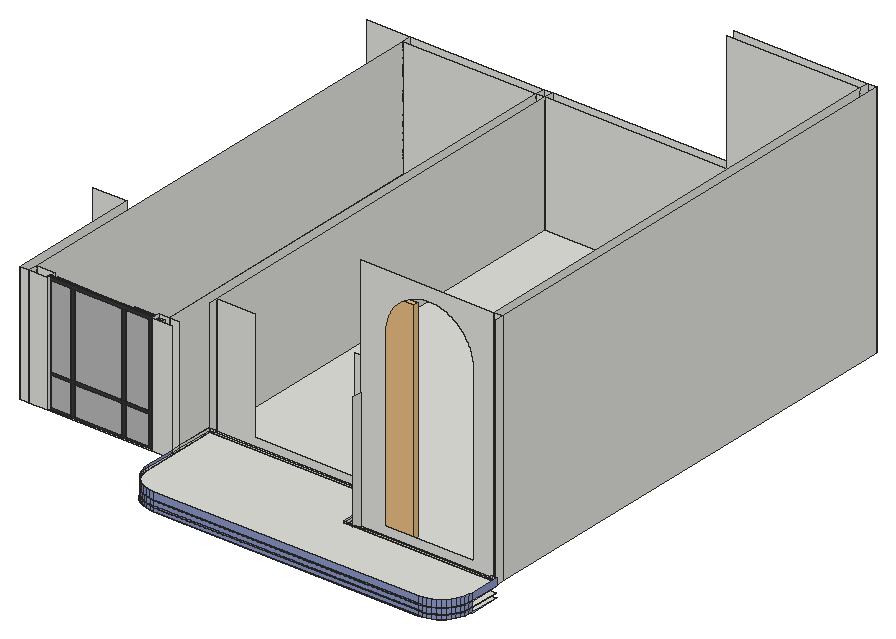
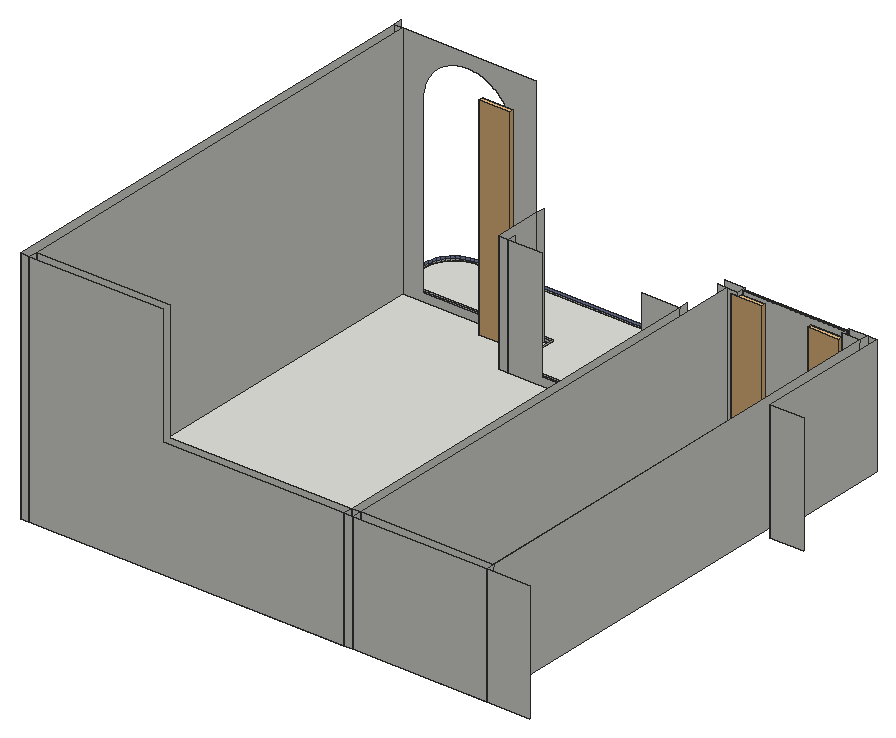
# SketchUp Ruby script. Lengths in inches.
U = 1.inch
M = Sketchup.active_model
def pt(a) = Geom::Point3d.new(a.map { |v| v * U })
def face(e, loops, mat)
  f = e.add_face(loops[0].map { |a| pt(a) })
  loops[1..].each { |l| e.add_face(l.map { |a| pt(a) }).erase! }
  f.material = f.back_material = mat if mat
  f
end
# faces: each face lists its corners as indices into pts; further lists are holes
def faces(e, pts, list, mat = nil) = list.each { |f| face(e, (f[0].is_a?(Array) ? f : [f]).map { |l| l.map { |i| pts[i] } }, mat) }
# xy, xz, yz: faces in a plane at the given z, y or x. An outline is a flat list of corners, or four numbers for a rectangle; further outlines are holes
def ring(l) = l.size == 4 ? [[l[0], l[1]], [l[2], l[1]], [l[2], l[3]], [l[0], l[3]]] : l.each_slice(2).to_a
def flat(e, list, mat, &to3) = list.each { |f| face(e, (f[0].is_a?(Array) ? f : [f]).map { |l| ring(l).map { |u, v| to3.(u, v) } }, mat) }
def xy(e, z, list, mat = nil) = flat(e, list, mat) { |x, y| [x, y, z] }
def xz(e, y, list, mat = nil) = flat(e, list, mat) { |x, z| [x, y, z] }
def yz(e, x, list, mat = nil) = flat(e, list, mat) { |y, z| [x, y, z] }
def lines(e, pts, list) = list.each { |a, b| e.add_line(pt(pts[a]), pt(pts[b])) }
# prism: a flat outline (further loops are holes) pulled along v
def prism(e, loops, v, mat = nil)
  f = face(e, loops, mat); d = Geom::Vector3d.new(v.map { |x| x * U })
  f.pushpull(f.normal.samedirection?(d) ? d.length : -d.length)
end
def box(e, o, s, mat = nil) = prism(e, [[o, [o[0] + s[0], o[1], o[2]], [o[0] + s[0], o[1] + s[1], o[2]], [o[0], o[1] + s[1], o[2]]]], [0, 0, s[2]], mat)
def at(x, y, z, deg = 0) = Geom::Transformation.translation(pt([x, y, z])) * Geom::Transformation.rotation(ORIGIN, Z_AXIS, deg.degrees)
def axes(o, x, y, z) = Geom::Transformation.new([*x, 0, *y, 0, *z, 0, *pt(o).to_a, 1])
def part(name) = M.definitions.add(name)
# library, detail: a bought-in or finely detailed component or shape, given as its bounding box
def library(name, o, s) = part(name).tap { |d| box(d.entities, o, s) }
def detail(e, o, s) = box(e.add_group.entities, o, s)
def put(e, d, t, mat = nil) = e.add_instance(d, t).tap { |i| i.material = mat if mat }
def group(e, t, mat = nil) = e.add_group.tap { |g| g.transformation = t; g.material = mat if mat }.entities
root = M.entities
M.materials.add("0326 AP 7207 CLASSIC PURPLE").color = [140, 152, 201]
M.materials.add("[Color M07]").color = [58, 58, 58]
M.materials.add("[Mirror 01]").color = [185, 185, 185]
c1 = library("Curtains 004",[-15.59,-2.26,0],[31.18,4.52,116.91])
xy(root,120.625,[[220.41,30.14,217,30.36,213.65,31.03,210.41,32.125,207.35,33.64,204.51,35.53,201.94,37.79,199.69,40.35,197.79,43.19,196.28,46.26,195.18,49.49,194.52,52.84,194.29,56.25,194.29,109.85,196.02,109.85,196.02,56.25,196.23,53.07,196.85,49.9375,197.88,46.92,199.29,44.06,201.0625,41.41,203.16,39.01,205.5625,36.9,208.21,35.13,211.08,33.72,214.1,32.7,217.22,32.07,220.41,31.87,487.22,31.87,490.59,32.09,493.71,32.71,496.73,33.73,499.59,35.14,502.24,36.91,504.64,39.02,506.74,41.41,508.51,44.0625,509.92,46.92,510.95,49.94,511.57,53.07,511.79,56.43,511.79,86.25,513.52,86.25,513.52,56.38,513.29,52.84,512.62,49.49,511.52,46.26,510.01,43.2,508.12,40.36,505.87,37.79,505.84,37.77,503.3,35.54,500.46,33.64,497.4,32.13,494.16,31.03,490.8125,30.37,487.28,30.14]])
xy(root,120.9375,[[220.41,29.57,216.92,29.79,213.5,30.47,210.2,31.6,207.06,33.14,204.16,35.08,201.54,37.38,199.24,40.01,197.3,42.91,195.75,46.04,194.63,49.34,193.95,52.77,193.72,56.25,193.72,109.85,196.02,109.85,196.02,56.25,196.23,53.07,196.85,49.9375,197.88,46.92,199.29,44.06,201.0625,41.41,203.16,39.01,205.5625,36.9,208.21,35.13,211.08,33.72,214.1,32.7,217.22,32.07,220.41,31.87,487.22,31.87,490.59,32.09,493.71,32.71,496.73,33.73,499.59,35.14,502.24,36.91,504.64,39.02,506.74,41.41,508.51,44.0625,509.92,46.92,510.95,49.94,511.57,53.07,511.79,56.43,511.79,86.25,514.09,86.25,514.09,56.36,513.86,52.77,513.18,49.35,512.05,46.04,510.51,42.91,508.57,40.01,506.27,37.39,506.22,37.34,503.65,35.09,500.75,33.15,497.62,31.6,494.3125,30.48,490.89,29.8,487.3,29.57]])
xy(root,121.1875,[[220.41,26.25,487.41,26.25,491.32,26.51,495.17,27.27,498.89,28.53,502.41,30.27,505.67,32.45,508.41,34.85,508.62,35.04,511.21,37.99,513.39,41.25,515.125,44.77,516.38,48.49,517.15,52.33,517.41,56.25,517.41,86.25,364.41,86.25,364.41,133.75,190.41,133.75,190.41,56.25,190.66,52.33,191.43,48.49,192.69,44.77,194.43,41.25,196.61,37.99,199.19,35.04,202.14,32.45,205.41,30.27,208.93,28.53,212.64,27.27,216.49,26.51]])
xy(root,121.1875,[[220.41,25.68,487.43,25.68,491.4,25.9375,495.32,26.72,499.11,28,502.69,29.77,506.02,32,508.78,34.42,509.02,34.63,511.66,37.64,513.88,40.96,515.65,44.55,516.9375,48.34,517.72,52.26,517.98,56.23,517.98,86.82,517.41,86.82,517.41,56.25,517.15,52.33,516.38,48.49,515.125,44.77,513.39,41.25,511.21,37.99,508.62,35.04,508.41,34.85,505.67,32.45,502.41,30.27,498.89,28.53,495.17,27.27,491.32,26.51,487.41,26.25,220.41,26.25,216.49,26.51,212.64,27.27,208.93,28.53,205.41,30.27,202.14,32.45,199.19,35.04,196.61,37.99,194.43,41.25,192.69,44.77,191.43,48.49,190.66,52.33,190.41,56.25,190.41,86.25,189.84,86.25,189.84,56.25,190.1,52.26,190.88,48.34,192.16,44.55,193.93,40.96,196.15,37.64,198.79,34.63,201.8,32,205.12,29.77,208.71,28.01,212.49,26.72,216.42,25.94]],"0326 AP 7207 CLASSIC PURPLE")
xy(root,124.75,[[220.41,26.25,487.41,26.25,491.32,26.51,495.17,27.27,498.89,28.53,502.41,30.27,505.67,32.45,508.62,35.04,511.21,37.99,513.39,41.25,515.125,44.77,516.38,48.49,517.15,52.33,517.41,56.25,517.41,86.25,364.41,86.25,364.41,133.75,190.41,133.75,190.41,56.25,190.66,52.33,191.43,48.49,192.69,44.77,194.43,41.25,196.61,37.99,199.19,35.04,202.14,32.45,205.41,30.27,208.93,28.53,212.64,27.27,216.49,26.51]])
xy(root,125.8125,[[220.41,26.25,487.41,26.25,491.32,26.51,495.17,27.27,498.89,28.53,502.41,30.27,505.67,32.45,508.62,35.04,511.21,37.99,513.39,41.25,515.125,44.77,516.38,48.49,517.15,52.33,517.41,56.25,517.41,86.25,364.41,86.25,364.41,133.75,190.41,133.75,190.41,56.25,190.66,52.33,191.43,48.49,192.69,44.77,194.43,41.25,196.61,37.99,199.19,35.04,202.14,32.45,205.41,30.27,208.93,28.53,212.64,27.27,216.49,26.51]])
xy(root,130.64,[[63.57,88.4,168.59,90.22]],"[Color M07]")
xy(root,130.9375,[[220.41,26.25,487.41,26.25,491.32,26.51,495.17,27.27,498.89,28.53,502.41,30.27,505.67,32.45,508.62,35.04,511.21,37.99,513.39,41.25,515.125,44.77,516.38,48.49,517.15,52.33,517.41,56.25,517.41,86.25,364.41,86.25,364.41,133.75,190.41,133.75,190.41,56.25,190.66,52.33,191.43,48.49,192.69,44.77,194.43,41.25,196.61,37.99,199.19,35.04,202.14,32.45,205.41,30.27,208.93,28.53,212.64,27.27,216.49,26.51]])
xy(root,132,[[46.41,86.25,65.51,95.25],[65.51,86.25,169.65,95.25],[169.65,86.25,190.41,95.25],[364.41,86.25,373.41,142.75],[373.41,86.25,517.41,95.25],
  [46.41,95.25,181.41,557.25],[181.41,95.25,190.41,557.25],[373.41,95.25,508.41,95.25,508.41,557.25,190.41,557.25,190.41,142.75,373.41,142.75],[508.41,95.25,517.41,566.25],[190.41,133.75,364.41,142.75],
  [46.41,557.25,181.41,566.25],[181.41,557.25,190.41,566.25],[190.41,557.25,508.41,566.25]])
xy(root,132.125,[[220.41,25.95,216.45,26.21,212.5625,26.98,208.81,28.25,205.26,30.01,201.96,32.21,198.98,34.82,196.37,37.8,194.16,41.1,192.41,44.65,191.14,48.41,190.36,52.29,190.1,56.25,190.1,134.05,195.11,134.05,195.11,133.75,190.41,133.75,190.41,56.25,190.66,52.33,191.43,48.49,192.69,44.77,194.43,41.25,196.61,37.99,199.19,35.04,202.14,32.45,205.41,30.27,208.93,28.53,212.64,27.27,216.49,26.51,220.41,26.25,487.41,26.25,491.32,26.51,495.17,27.27,498.89,28.53,502.41,30.27,505.67,32.45,508.62,35.04,511.21,37.99,513.39,41.25,515.125,44.77,516.38,48.49,517.15,52.33,517.41,56.25,517.41,86.25,512.71,86.25,512.71,86.55,517.71,86.55,517.71,56.25,517.45,52.29,516.68,48.41,515.4,44.65,513.65,41.1,511.45,37.8,508.83,34.82,505.85,32.21,502.56,30.01,499,28.25,495.25,26.98,491.36,26.21,487.41,25.95]],"0326 AP 7207 CLASSIC PURPLE")
xy(root,132.1875,[[220.41,26.25,487.41,26.25,491.32,26.51,495.17,27.27,498.89,28.53,502.41,30.27,505.67,32.45,508.62,35.04,511.21,37.99,513.39,41.25,515.125,44.77,516.38,48.49,517.15,52.33,517.41,56.25,517.41,86.25,364.41,86.25,364.41,133.75,190.41,133.75,190.41,56.25,190.66,52.33,191.43,48.49,192.69,44.77,194.43,41.25,196.61,37.99,199.19,35.04,202.14,32.45,205.41,30.27,208.93,28.53,212.64,27.27,216.49,26.51]])
xy(root,133.36,[[66.28,88.4,86.85,88.84],[90.47,88.4,138.0625,88.84],[142.18,88.4,165.87,88.84]],"[Color M07]")
xy(root,135.3125,[[220.41,26.25,487.41,26.25,491.32,26.51,495.17,27.27,498.89,28.53,502.41,30.27,505.67,32.45,508.62,35.04,511.21,37.99,513.39,41.25,515.125,44.77,516.38,48.49,517.15,52.33,517.41,56.25,517.41,86.25,364.41,86.25,364.41,133.75,190.41,133.75,190.41,56.25,190.66,52.33,191.43,48.49,192.69,44.77,194.43,41.25,196.61,37.99,199.19,35.04,202.14,32.45,205.41,30.27,208.93,28.53,212.64,27.27,216.49,26.51]])
xy(root,163.14,[[66.28,88.4,86.85,88.84],[90.47,88.4,138.0625,88.84],[142.18,88.4,165.87,88.84]],"[Color M07]")
xy(root,165.91,[[66.28,88.4,86.85,88.84],[90.47,88.4,138.0625,88.84],[142.18,88.4,165.87,88.84]],"[Color M07]")
xy(root,248.8,[[66.28,88.4,86.85,88.84],[90.47,88.4,138.0625,88.84],[142.18,88.4,165.87,88.84]],"[Color M07]")
xy(root,251.52,[[63.57,88.4,168.59,90.22]],"[Color M07]")
xz(root,25.95,[[220.41,132.125,487.41,139.125]],"0326 AP 7207 CLASSIC PURPLE")
xz(root,26.25,[[220.41,132.125,487.41,132.1875],[220.41,132.1875,487.41,135.3125],[220.41,135.3125,487.41,136.75]])
xz(root,26.25,[[220.41,121.1875,487.41,124.75],[220.41,124.75,487.41,125.8125],[220.41,125.8125,487.41,130.9375],[220.41,130.9375,487.41,132.125]],"0326 AP 7207 CLASSIC PURPLE")
xz(root,31.87,[[220.41,120.625,487.22,120.9375]])
xz(root,86.25,[[37.41,132,46.41,252],[46.41,132,65.51,252],[169.65,132,190.41,252],[364.41,132,373.41,132.1875],[373.41,132,398.23,132.1875],
  [398.23,132,487.79,132.1875],[487.79,132,517.41,132,517.41,132.125,512.71,132.125,512.71,132.1875,487.79,132.1875],[512.71,132.125,513.01,132.1875],[513.01,132.125,517.41,132.1875],[364.41,132.1875,373.41,135.3125],
  [373.41,132.1875,398.23,135.3125],[398.23,132.1875,487.79,135.3125],[487.79,132.1875,512.71,135.3125],[512.71,132.1875,513.01,135.3125],[513.01,132.1875,517.41,135.3125],
  [364.41,135.3125,373.41,136.75],[373.41,135.3125,398.23,136.75],[398.23,135.3125,487.79,136.75],[487.79,135.3125,512.71,136.75],[512.71,135.3125,513.01,136.75],
  [513.01,135.3125,517.41,136.75]])
xz(root,86.55,[[512.71,132.125,517.71,139.125]])
xz(root,88.4,[[[63.57,130.64,168.59,251.52],[66.28,133.36,165.87,248.8]],[86.85,133.36,90.47,163.14],[138.0625,133.36,142.18,163.14],[66.28,163.14,86.85,165.91],[86.85,163.14,90.47,165.91],
  [90.47,163.14,138.0625,165.91],[138.0625,163.14,142.18,165.91],[142.18,163.14,165.87,165.91],[86.85,165.91,90.47,248.8],[138.0625,165.91,142.18,248.8]],"[Color M07]")
xz(root,88.84,[[66.28,133.36,86.85,163.14],[90.47,133.36,138.0625,163.14],[142.18,133.36,165.87,163.14],[66.28,165.91,86.85,248.8],[90.47,165.91,138.0625,248.8],
  [142.18,165.91,165.87,248.8]],"[Mirror 01]")
xz(root,90.22,[[63.57,130.64,168.59,251.52]])
xz(root,95.25,[[46.41,132,65.51,252],[169.65,132,181.41,252],[181.41,132,190.41,252],[[373.41,132,508.41,372],[398.23,140.0625,487.79,140.0625,487.79,316.97,487.68,318.34,487.51,319.8,487.3,321.26,487.04,322.7,486.73,324.14,486.375,325.57,485.97,326.98,485.52,328.38,485.03,329.77,484.49,331.13,483.91,332.48,483.28,333.8125,482.61,335.12,481.9,336.41,481.14,337.67,480.35,338.9,479.51,340.11,478.64,341.29,477.72,342.44,476.77,343.57,475.79,344.66,474.77,345.71,473.71,346.74,472.62,347.72,471.5,348.67,470.35,349.59,469.17,350.47,467.96,351.3,466.73,352.1,465.47,352.86,464.18,353.57,462.875,354.24,461.55,354.87,460.2,355.46,458.83,356,457.45,356.49,456.05,356.94,454.64,357.35,453.21,357.7,451.77,358.01,450.33,358.28,448.87,358.49,447.41,358.66,445.95,358.78,444.48,358.85,443.01,358.88,441.54,358.85,440.07,358.78,438.61,358.66,437.15,358.49,435.69,358.28,434.25,358.01,432.8125,357.7,431.38,357.35,429.97,356.94,428.57,356.49,427.1875,356,425.82,355.46,424.47,354.87,423.14,354.24,421.84,353.57,420.55,352.86,419.29,352.1,418.06,351.3,416.85,350.47,415.67,349.59,414.52,348.67,413.4,347.72,412.31,346.74,411.25,345.71,410.23,344.66,409.25,343.57,408.3,342.44,407.38,341.29,406.51,340.11,405.67,338.9,404.88,337.67,404.125,336.41,403.41,335.12,402.74,333.8125,402.11,332.48,401.53,331.13,400.99,329.77,400.5,328.38,400.05,326.98,399.65,325.57,399.29,324.14,398.98,322.7,398.72,321.26,398.51,319.8,398.34,318.34,398.23,316.97]],[508.41,132,517.41,372]])
xz(root,133.75,[[190.41,132,364.41,132,364.41,132.1875,195.11,132.1875,195.11,132.125,190.41,132.125],[190.41,132.125,194.8,132.1875],[194.8,132.125,195.11,132.1875],[190.41,132.1875,194.8,135.3125],[194.8,132.1875,195.11,135.3125],
  [195.11,132.1875,364.41,135.3125],[190.41,135.3125,194.8,136.75],[194.8,135.3125,195.11,136.75],[195.11,135.3125,364.41,136.75]])
xz(root,134.05,[[190.1,132.125,195.11,139.125]])
xz(root,142.75,[[190.41,132,190.41,252,228.58,252,228.58,140.0625,330.09,140.0625,330.09,252,364.41,252,364.41,132],[364.41,132,373.41,252]])
xz(root,220.92,[[2.97,132,37.41,252]])
xz(root,557.25,[[46.41,132,181.41,252],[181.41,132,190.41,252],[190.41,132,508.41,132,508.41,372,373.41,372,373.41,252,190.41,252]])
xz(root,566.25,[[2.97,132,46.41,252],[46.41,132,181.41,252],[181.41,132,190.41,252],[190.41,132,190.41,252,373.41,252,373.41,372,508.41,372,508.41,132],[508.41,132,517.41,372]])
yz(root,37.41,[[86.25,132,220.92,252]])
yz(root,46.41,[[86.25,132,95.25,252],[95.25,132,557.25,252],[557.25,132,566.25,252]])
yz(root,63.57,[[88.4,130.64,90.22,251.52]],"[Color M07]")
yz(root,65.51,[[86.25,132,95.25,252]])
yz(root,66.28,[[88.4,133.36,88.84,163.14]])
yz(root,66.28,[[88.4,165.91,88.84,248.8]],"[Color M07]")
yz(root,86.85,[[88.4,133.36,88.84,163.14],[88.4,165.91,88.84,248.8]],"[Color M07]")
yz(root,90.47,[[88.4,133.36,88.84,163.14]])
yz(root,90.47,[[88.4,165.91,88.84,248.8]],"[Color M07]")
yz(root,138.0625,[[88.4,133.36,88.84,163.14],[88.4,165.91,88.84,248.8]],"[Color M07]")
yz(root,142.18,[[88.4,133.36,88.84,163.14]])
yz(root,142.18,[[88.4,165.91,88.84,248.8]],"[Color M07]")
yz(root,165.87,[[88.4,133.36,88.84,163.14],[88.4,165.91,88.84,248.8]],"[Color M07]")
yz(root,168.59,[[88.4,130.64,90.22,251.52]],"[Color M07]")
yz(root,169.65,[[86.25,132,95.25,252]])
yz(root,181.41,[[95.25,132,557.25,252],[557.25,132,566.25,252]])
yz(root,190.1,[[86.25,132.125,95.25,139.125],[95.25,132.125,134.05,139.125]])
yz(root,190.1,[[56.25,132.125,86.25,139.125]],"0326 AP 7207 CLASSIC PURPLE")
yz(root,190.41,[[86.25,132,95.25,132.125],[95.25,132,133.75,132.125],[133.75,132,142.75,252],[142.75,132,557.25,252],[557.25,132,566.25,252],
  [56.25,132.125,86.25,132.1875],[86.25,132.125,95.25,132.1875],[95.25,132.125,133.75,132.1875],[56.25,132.1875,86.25,135.3125],[86.25,132.1875,95.25,135.3125],
  [95.25,132.1875,133.75,135.3125],[56.25,135.3125,86.25,136.75],[86.25,135.3125,95.25,136.75],[95.25,135.3125,133.75,136.75]])
yz(root,190.41,[[56.25,121.1875,86.25,124.75],[56.25,124.75,86.25,125.8125],[56.25,125.8125,86.25,130.9375],[56.25,130.9375,86.25,132.125]],"0326 AP 7207 CLASSIC PURPLE")
yz(root,195.11,[[133.75,132.125,134.05,139.125]])
yz(root,196.02,[[56.25,120.625,86.25,120.9375],[86.25,120.625,109.85,120.9375]])
yz(root,364.41,[[86.25,132,133.75,132.1875],[133.75,132,142.75,252],[86.25,132.1875,133.75,135.3125],[86.25,135.3125,133.75,136.75]])
yz(root,373.41,[[86.25,132,95.25,252],[95.25,132,142.75,252]])
yz(root,508.41,[[95.25,132,557.25,372],[557.25,132,566.25,372]])
yz(root,511.79,[[56.43,120.625,86.25,120.9375]])
yz(root,512.71,[[86.25,132.125,86.55,139.125]])
yz(root,517.41,[[86.25,132,95.25,372],[95.25,132,566.25,372],[56.25,132.125,86.25,132.1875],[56.25,132.1875,86.25,135.3125],[56.25,135.3125,86.25,136.75]])
yz(root,517.71,[[56.25,132.125,86.55,139.125]],"0326 AP 7207 CLASSIC PURPLE")
p = [[217.22,32.07,120.9375],[217.22,32.07,120.625],[220.41,31.87,120.625],[220.41,31.87,120.9375],[487.22,31.87,120.9375],[487.22,31.87,120.625],
  [490.59,32.09,120.625],[490.59,32.09,120.9375],[214.1,32.7,120.9375],[214.1,32.7,120.625],[493.71,32.71,120.625],[493.71,32.71,120.9375],
  [211.08,33.72,120.9375],[211.08,33.72,120.625],[496.73,33.73,120.625],[496.73,33.73,120.9375],[208.21,35.13,120.9375],[208.21,35.13,120.625],
  [499.59,35.14,120.625],[499.59,35.14,120.9375],[205.5625,36.9,120.9375],[205.5625,36.9,120.625],[502.24,36.91,120.625],[502.24,36.91,120.9375],
  [203.16,39.01,120.9375],[203.16,39.01,120.625],[504.64,39.02,120.625],[504.64,39.02,120.9375],[201.0625,41.41,120.9375],[201.0625,41.41,120.625],
  [506.74,41.41,120.625],[506.74,41.41,120.9375],[199.29,44.06,120.9375],[199.29,44.06,120.625],[508.51,44.0625,120.625],[508.51,44.0625,120.9375],
  [197.88,46.92,120.9375],[197.88,46.92,120.625],[509.92,46.92,120.625],[509.92,46.92,120.9375],[196.85,49.9375,120.9375],[196.85,49.9375,120.625],
  [510.95,49.94,120.625],[510.95,49.94,120.9375],[196.23,53.07,120.9375],[196.23,53.07,120.625],[511.57,53.07,120.625],[511.57,53.07,120.9375],
  [196.02,56.25,120.9375],[196.02,56.25,120.625],[511.79,56.43,120.625],[511.79,56.43,120.9375],[216.49,26.51,124.75],[216.49,26.51,121.1875],
  [220.41,26.25,121.1875],[220.41,26.25,124.75],[487.41,26.25,124.75],[487.41,26.25,121.1875],[491.32,26.51,121.1875],[491.32,26.51,124.75],
  [212.64,27.27,124.75],[212.64,27.27,121.1875],[495.17,27.27,121.1875],[495.17,27.27,124.75],[208.93,28.53,124.75],[208.93,28.53,121.1875],
  [498.89,28.53,121.1875],[498.89,28.53,124.75],[205.41,30.27,124.75],[205.41,30.27,121.1875],[502.41,30.27,121.1875],[502.41,30.27,124.75],
  [202.14,32.45,124.75],[202.14,32.45,121.1875],[505.67,32.45,121.1875],[505.67,32.45,124.75],[199.19,35.04,124.75],[199.19,35.04,121.1875],
  [508.41,34.85,121.1875],[508.62,35.04,121.1875],[508.62,35.04,124.75],[196.61,37.99,124.75],[196.61,37.99,121.1875],[511.21,37.99,121.1875],
  [511.21,37.99,124.75],[194.43,41.25,124.75],[194.43,41.25,121.1875],[513.39,41.25,121.1875],[513.39,41.25,124.75],[192.69,44.77,124.75],
  [192.69,44.77,121.1875],[515.125,44.77,121.1875],[515.125,44.77,124.75],[191.43,48.49,124.75],[191.43,48.49,121.1875],[516.38,48.49,121.1875],
  [516.38,48.49,124.75],[190.66,52.33,124.75],[190.66,52.33,121.1875],[517.15,52.33,121.1875],[517.15,52.33,124.75],[190.41,56.25,124.75],
  [190.41,56.25,121.1875],[517.41,56.25,121.1875],[517.41,56.25,124.75],[216.49,26.51,125.8125],[220.41,26.25,125.8125],[487.41,26.25,125.8125],
  [491.32,26.51,125.8125],[212.64,27.27,125.8125],[495.17,27.27,125.8125],[208.93,28.53,125.8125],[498.89,28.53,125.8125],[205.41,30.27,125.8125],
  [502.41,30.27,125.8125],[202.14,32.45,125.8125],[505.67,32.45,125.8125],[199.19,35.04,125.8125],[508.62,35.04,125.8125],[196.61,37.99,125.8125],
  [511.21,37.99,125.8125],[194.43,41.25,125.8125],[513.39,41.25,125.8125],[192.69,44.77,125.8125],[515.125,44.77,125.8125],[191.43,48.49,125.8125],
  [516.38,48.49,125.8125],[190.66,52.33,125.8125],[517.15,52.33,125.8125],[190.41,56.25,125.8125],[517.41,56.25,125.8125],[216.49,26.51,130.9375],
  [220.41,26.25,130.9375],[487.41,26.25,130.9375],[491.32,26.51,130.9375],[212.64,27.27,130.9375],[495.17,27.27,130.9375],[208.93,28.53,130.9375],
  [498.89,28.53,130.9375],[205.41,30.27,130.9375],[502.41,30.27,130.9375],[202.14,32.45,130.9375],[505.67,32.45,130.9375],[199.19,35.04,130.9375],
  [508.62,35.04,130.9375],[196.61,37.99,130.9375],[511.21,37.99,130.9375],[194.43,41.25,130.9375],[513.39,41.25,130.9375],[192.69,44.77,130.9375],
  [515.125,44.77,130.9375],[191.43,48.49,130.9375],[516.38,48.49,130.9375],[190.66,52.33,130.9375],[517.15,52.33,130.9375],[190.41,56.25,130.9375],
  [517.41,56.25,130.9375],[220.41,26.25,132.125],[216.49,26.51,132.125],[491.32,26.51,132.125],[487.41,26.25,132.125],[212.64,27.27,132.125],
  [495.17,27.27,132.125],[208.93,28.53,132.125],[498.89,28.53,132.125],[205.41,30.27,132.125],[502.41,30.27,132.125],[202.14,32.45,132.125],
  [505.67,32.45,132.125],[199.19,35.04,132.125],[508.62,35.04,132.125],[196.61,37.99,132.125],[511.21,37.99,132.125],[194.43,41.25,132.125],
  [513.39,41.25,132.125],[192.69,44.77,132.125],[515.125,44.77,132.125],[191.43,48.49,132.125],[516.38,48.49,132.125],[190.66,52.33,132.125],
  [517.15,52.33,132.125],[190.41,56.25,132.125],[517.41,56.25,132.125],[220.41,25.95,139.125],[216.45,26.21,139.125],[216.45,26.21,132.125],
  [220.41,25.95,132.125],[491.36,26.21,139.125],[487.41,25.95,139.125],[487.41,25.95,132.125],[491.36,26.21,132.125],[212.5625,26.98,139.125],
  [212.5625,26.98,132.125],[216.49,26.51,132.1875],[220.41,26.25,132.1875],[487.41,26.25,132.1875],[491.32,26.51,132.1875],[495.25,26.98,139.125],
  [495.25,26.98,132.125],[212.64,27.27,132.1875],[495.17,27.27,132.1875],[208.81,28.25,139.125],[208.81,28.25,132.125],[499,28.25,139.125],
  [499,28.25,132.125],[208.93,28.53,132.1875],[498.89,28.53,132.1875],[205.26,30.01,139.125],[205.26,30.01,132.125],[502.56,30.01,139.125],
  [502.56,30.01,132.125],[205.41,30.27,132.1875],[502.41,30.27,132.1875],[201.96,32.21,139.125],[201.96,32.21,132.125],[505.85,32.21,139.125],
  [505.85,32.21,132.125],[202.14,32.45,132.1875],[505.67,32.45,132.1875],[198.98,34.82,139.125],[198.98,34.82,132.125],[508.83,34.82,139.125],
  [508.83,34.82,132.125],[199.19,35.04,132.1875],[508.62,35.04,132.1875],[196.37,37.8,139.125],[196.37,37.8,132.125],[511.45,37.8,139.125],
  [511.45,37.8,132.125],[196.61,37.99,132.1875],[511.21,37.99,132.1875],[194.16,41.1,139.125],[194.16,41.1,132.125],[513.65,41.1,139.125],
  [513.65,41.1,132.125],[194.43,41.25,132.1875],[513.39,41.25,132.1875],[192.41,44.65,139.125],[192.41,44.65,132.125],[515.4,44.65,139.125],
  [515.4,44.65,132.125],[192.69,44.77,132.1875],[515.125,44.77,132.1875],[191.14,48.41,139.125],[191.14,48.41,132.125],[516.68,48.41,139.125],
  [516.68,48.41,132.125],[191.43,48.49,132.1875],[516.38,48.49,132.1875],[190.36,52.29,139.125],[190.36,52.29,132.125],[517.45,52.29,139.125],
  [517.45,52.29,132.125],[190.66,52.33,132.1875],[517.15,52.33,132.1875],[190.1,56.25,139.125],[190.1,56.25,132.125],[190.41,56.25,132.1875],
  [517.41,56.25,132.1875],[517.71,56.25,139.125],[517.71,56.25,132.125],[216.49,26.51,135.3125],[220.41,26.25,135.3125],[487.41,26.25,135.3125],
  [491.32,26.51,135.3125],[212.64,27.27,135.3125],[495.17,27.27,135.3125],[208.93,28.53,135.3125],[498.89,28.53,135.3125],[205.41,30.27,135.3125],
  [502.41,30.27,135.3125],[202.14,32.45,135.3125],[505.67,32.45,135.3125],[199.19,35.04,135.3125],[508.62,35.04,135.3125],[196.61,37.99,135.3125],
  [511.21,37.99,135.3125],[194.43,41.25,135.3125],[513.39,41.25,135.3125],[192.69,44.77,135.3125],[515.125,44.77,135.3125],[191.43,48.49,135.3125],
  [516.38,48.49,135.3125],[190.66,52.33,135.3125],[517.15,52.33,135.3125],[190.41,56.25,135.3125],[517.41,56.25,135.3125],[216.49,26.51,136.75],
  [220.41,26.25,136.75],[487.41,26.25,136.75],[491.32,26.51,136.75],[212.64,27.27,136.75],[495.17,27.27,136.75],[208.93,28.53,136.75],
  [498.89,28.53,136.75],[205.41,30.27,136.75],[502.41,30.27,136.75],[202.14,32.45,136.75],[505.67,32.45,136.75],[199.19,35.04,136.75],
  [508.62,35.04,136.75],[196.61,37.99,136.75],[511.21,37.99,136.75],[194.43,41.25,136.75],[513.39,41.25,136.75],[192.69,44.77,136.75],
  [515.125,44.77,136.75],[191.43,48.49,136.75],[516.38,48.49,136.75],[190.66,52.33,136.75],[517.15,52.33,136.75],[190.41,56.25,136.75],
  [517.41,56.25,136.75]]
faces(root,p,[[0,1,2,3],[4,5,6,7],[8,9,1,0],[7,6,10,11],[12,13,9,8],[11,10,14,15],[16,17,13,12],[15,14,18,19],
  [20,21,17,16],[19,18,22,23],[24,25,21,20],[23,22,26,27],[28,29,25,24],[27,26,30,31],[32,33,29,28],[31,30,34,35],
  [36,37,33,32],[35,34,38,39],[40,41,37,36],[39,38,42,43],[44,45,41,40],[43,42,46,47],[48,49,45,44],[47,46,50,51],
  [158,193,194,157],[195,160,159,196],[161,199,193,158],[159,196,200,162],[163,205,199,161],[162,200,206,164],[165,211,205,163],[164,206,212,166],
  [167,217,211,165],[166,212,218,168],[169,223,217,167],[168,218,224,170],[171,229,223,169],[170,224,230,172],[173,235,229,171],[172,230,236,174],
  [175,241,235,173],[174,236,242,176],[177,247,241,175],[176,242,248,178],[253,179,177,247],[178,248,254,180],[257,181,179,253],[254,180,182,258],
  [261,193,194,262],[195,263,264,196],[265,199,193,261],[264,196,200,266],[267,205,199,265],[266,200,206,268],[269,211,205,267],[268,206,212,270],
  [271,217,211,269],[270,212,218,272],[273,223,217,271],[272,218,224,274],[275,229,223,273],[274,224,230,276],[277,235,229,275],[276,230,236,278],
  [279,241,235,277],[278,236,242,280],[281,247,241,279],[280,242,248,282],[253,283,281,247],[282,248,254,284],[257,285,283,253],[254,284,286,258],
  [261,287,288,262],[263,289,290,264],[265,291,287,261],[264,290,292,266],[267,293,291,265],[266,292,294,268],[269,295,293,267],[268,294,296,270],
  [271,297,295,269],[270,296,298,272],[273,299,297,271],[272,298,300,274],[275,301,299,273],[274,300,302,276],[277,303,301,275],[276,302,304,278],
  [279,305,303,277],[278,304,306,280],[281,307,305,279],[280,306,308,282],[283,309,307,281],[282,308,310,284],[285,311,309,283],[284,310,312,286]])
faces(root,p,[[52,53,54,55],[56,57,58,59],[60,61,53,52],[59,58,62,63],[64,65,61,60],[63,62,66,67],[68,69,65,64],[67,66,70,71],
  [72,73,69,68],[71,70,74,75],[76,77,73,72],[75,74,78,79,80],[81,82,77,76],[80,79,83,84],[85,86,82,81],[84,83,87,88],
  [89,90,86,85],[88,87,91,92],[93,94,90,89],[92,91,95,96],[97,98,94,93],[96,95,99,100],[101,102,98,97],[100,99,103,104],
  [105,52,55,106],[107,56,59,108],[109,60,52,105],[108,59,63,110],[111,64,60,109],[110,63,67,112],[113,68,64,111],[112,67,71,114],
  [115,72,68,113],[114,71,75,116],[117,76,72,115],[116,75,80,118],[119,81,76,117],[118,80,84,120],[121,85,81,119],[120,84,88,122],
  [123,89,85,121],[122,88,92,124],[125,93,89,123],[124,92,96,126],[127,97,93,125],[126,96,100,128],[129,101,97,127],[128,100,104,130],
  [131,105,106,132],[133,107,108,134],[135,109,105,131],[134,108,110,136],[137,111,109,135],[136,110,112,138],[139,113,111,137],[138,112,114,140],
  [141,115,113,139],[140,114,116,142],[143,117,115,141],[142,116,118,144],[145,119,117,143],[144,118,120,146],[147,121,119,145],[146,120,122,148],
  [149,123,121,147],[148,122,124,150],[151,125,123,149],[150,124,126,152],[153,127,125,151],[152,126,128,154],[155,129,127,153],[154,128,130,156],
  [132,157,158,131],[134,159,160,133],[131,158,161,135],[136,162,159,134],[135,161,163,137],[138,164,162,136],[137,163,165,139],[140,166,164,138],
  [139,165,167,141],[142,168,166,140],[141,167,169,143],[144,170,168,142],[143,169,171,145],[146,172,170,144],[145,171,173,147],[148,174,172,146],
  [147,173,175,149],[150,176,174,148],[149,175,177,151],[152,178,176,150],[151,177,179,153],[154,180,178,152],[153,179,181,155],[156,182,180,154],
  [183,184,185,186],[187,188,189,190],[184,191,192,185],[197,187,190,198],[191,201,202,192],[203,197,198,204],[201,207,208,202],[209,203,204,210],
  [207,213,214,208],[215,209,210,216],[213,219,220,214],[221,215,216,222],[219,225,226,220],[227,221,222,228],[225,231,232,226],[233,227,228,234],
  [231,237,238,232],[239,233,234,240],[237,243,244,238],[245,239,240,246],[243,249,250,244],[251,245,246,252],[249,255,256,250],[259,251,252,260]],"0326 AP 7207 CLASSIC PURPLE")
put(root,c1,axes([404.8,106.87,130.09],[1,0,0],[0,1,0],[0,0,1.83]))
put(root,c1,at(81.76,95.97,130.19))
put(root,c1,at(160.68,94.34,131.94))
